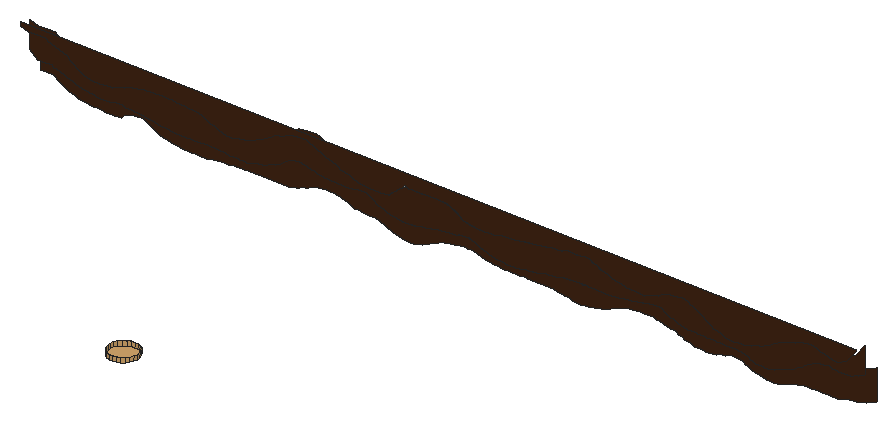
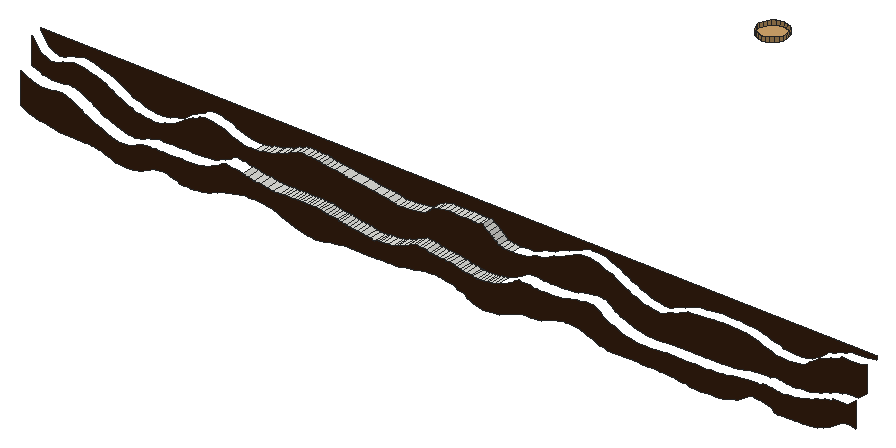
# SketchUp Ruby script. Lengths in inches.
U = 1.inch
M = Sketchup.active_model
def pt(a) = Geom::Point3d.new(a.map { |v| v * U })
def face(e, loops, mat)
  f = e.add_face(loops[0].map { |a| pt(a) })
  loops[1..].each { |l| e.add_face(l.map { |a| pt(a) }).erase! }
  f.material = f.back_material = mat if mat
  f
end
# faces: each face lists its corners as indices into pts; further lists are holes
def faces(e, pts, list, mat = nil) = list.each { |f| face(e, (f[0].is_a?(Array) ? f : [f]).map { |l| l.map { |i| pts[i] } }, mat) }
# xy, xz, yz: faces in a plane at the given z, y or x. An outline is a flat list of corners, or four numbers for a rectangle; further outlines are holes
def ring(l) = l.size == 4 ? [[l[0], l[1]], [l[2], l[1]], [l[2], l[3]], [l[0], l[3]]] : l.each_slice(2).to_a
def flat(e, list, mat, &to3) = list.each { |f| face(e, (f[0].is_a?(Array) ? f : [f]).map { |l| ring(l).map { |u, v| to3.(u, v) } }, mat) }
def xy(e, z, list, mat = nil) = flat(e, list, mat) { |x, y| [x, y, z] }
def xz(e, y, list, mat = nil) = flat(e, list, mat) { |x, z| [x, y, z] }
def yz(e, x, list, mat = nil) = flat(e, list, mat) { |y, z| [x, y, z] }
def lines(e, pts, list) = list.each { |a, b| e.add_line(pt(pts[a]), pt(pts[b])) }
# prism: a flat outline (further loops are holes) pulled along v
def prism(e, loops, v, mat = nil)
  f = face(e, loops, mat); d = Geom::Vector3d.new(v.map { |x| x * U })
  f.pushpull(f.normal.samedirection?(d) ? d.length : -d.length)
end
def box(e, o, s, mat = nil) = prism(e, [[o, [o[0] + s[0], o[1], o[2]], [o[0] + s[0], o[1] + s[1], o[2]], [o[0], o[1] + s[1], o[2]]]], [0, 0, s[2]], mat)
def at(x, y, z, deg = 0) = Geom::Transformation.translation(pt([x, y, z])) * Geom::Transformation.rotation(ORIGIN, Z_AXIS, deg.degrees)
def axes(o, x, y, z) = Geom::Transformation.new([*x, 0, *y, 0, *z, 0, *pt(o).to_a, 1])
def part(name) = M.definitions.add(name)
# library, detail: a bought-in or finely detailed component or shape, given as its bounding box
def library(name, o, s) = part(name).tap { |d| box(d.entities, o, s) }
def detail(e, o, s) = box(e.add_group.entities, o, s)
def put(e, d, t, mat = nil) = e.add_instance(d, t).tap { |i| i.material = mat if mat }
def group(e, t, mat = nil) = e.add_group.tap { |g| g.transformation = t; g.material = mat if mat }.entities
root = M.entities
M.materials.add("[Field Square Tile]").color = [211, 167, 108]
M.materials.add("[Wood Veneer 01]").color = [66, 38, 20]
xy(root,243.05,[[1237.04,563.18,1237.72,565.74]])
xy(root,243.07,[[1235.1875,563.18,1235.77,565.74]])
xy(root,243.09,[[1231.875,563.18,1232.4,565.74],[1232.4,563.18,1232.92,565.74],[1232.92,563.18,1233.58,565.74],[1233.58,563.18,1234.03,565.74]])
xy(root,249.21,[[1204.67,561.05,1205.56,563.18]])
xy(root,249.22,[[1206.28,561.05,1207.1875,563.18]])
xy(root,249.23,[[1207.83,561.05,1208.73,563.18]])
xy(root,250.6875,[[1203.22,492.77,1202.56,492.86,1201.94,493.11,1201.41,493.52,1201,494.05,1200.75,494.67,1200.66,495.33,1200.75,495.99,1201,496.61,1201.41,497.14,1201.94,497.55,1202.56,497.81,1203.22,497.89,1203.88,497.81,1204.5,497.55,1205.03,497.14,1205.44,496.61,1205.7,495.99,1205.78,495.33,1205.7,494.67,1205.44,494.05,1205.03,493.52,1204.5,493.11,1203.88,492.86]],"[Field Square Tile]")
xz(root,561.05,[[1263.09,244.87,1264,245.01,1264.9375,245.12,1265.7,245.25,1266.46,245.41,1267.09,245.78,1267.89,245.88,1268.6,246.16,1269.2,246.57,1269.99,246.9,1270.59,247.35,1271.26,247.62,1271.85,248.06,1272.61,248.32,1273.72,248.66,1274.5,248.79,1275.36,249.19,1276.03,249.32,1276.96,249.41,1277.81,249.48,1278.56,249.21,1279.2,248.96,1279.9,248.9,1280.7,248.42,1281.41,248.3,1282.12,248.22,1282.9375,248.56,1283.87,249.02,1285.6,251.16,1285.6,251.5,1131.59,251.5,1131.59,250.88,1133.18,250.53,1134.8,250.54,1136.26,250.55,1136.79,250.15,1137.4,249.97,1138.2,249.8,1138.87,249.41,1139.54,249.2,1140.31,249.01,1140.8,248.51,1141.43,248.07,1142.08,247.72,1142.72,247.25,1143.27,246.88,1143.99,246.73,1144.65,246.62,1145.39,246.54,1146.17,246.51,1146.95,246.58,1147.75,246.59,1148.55,246.69,1149.26,247.03,1149.95,247.2,1150.92,247.39,1151.55,247.78,1152.33,247.89,1153.33,248.18,1153.97,248.29,1154.86,248.35,1155.59,248.4,1156.58,248.4375,1157.24,248.46,1158.13,248.47,1158.87,248.48,1159.76,248.49,1160.49,248.39,1161.89,248.28,1162.92,248.15,1163.74,248.11,1164.54,248.08,1165.38,247.66,1166.01,247.46,1166.69,247.08,1167.375,246.94,1168.23,246.66,1168.84,246.35,1169.61,246.05,1170.51,246.13,1171.22,246.29,1172.02,246.41,1172.93,246.55,1173.66,246.92,1174.27,247.12,1174.95,247.31,1175.52,247.71,1176.45,248.03,1177.16,248.46,1177.94,248.82,1178.66,249.37,1179.45,249.5625,1180.35,249.9,1181.27,250.35,1181.93,250.49,1182.74,250.6,1183.76,250.58,1184.4,250.61,1185.02,250.32,1185.71,250.0625,1186.37,249.68,1187.13,249.46,1188.02,248.95,1189.24,248.69,1190.15,248.26,1190.75,247.9,1191.88,247.66,1192.46,247.53,1193.14,247.25,1193.95,246.95,1194.64,246.75,1195.43,246.66,1196.14,246.59,1197.03,246.55,1197.96,246.63,1198.7,246.74,1199.43,246.87,1200.04,247.42,1200.71,247.96,1201.28,248.44,1202.02,248.85,1202.49,249.34,1203.22,249.125,1203.99,249.17,1204.67,249.21,1205.56,249.21,1206.28,249.22,1207.1875,249.22,1207.83,249.23,1208.73,249.23,1209.47,249.24,1210.27,249.14,1210.9,248.82,1211.69,248.54,1212.39,248.04,1213.08,247.48,1213.97,247.29,1214.79,247.15,1215.52,247.05,1216.24,247,1217.15,246.96,1217.875,246.94,1218.79,247.04,1219.85,247.36,1221.03,247.43,1222.68,247.6,1224.66,247.98,1226.86,248.1875,1228.47,248.49,1229.72,248.62,1230.66,248.69,1231.34,248.75,1232,249.09,1232.7,249.18,1233.48,249.13,1234.18,249.17,1234.88,249.18,1235.78,249.29,1236.51,249.21,1237.12,248.8,1237.8125,248.73,1238.59,248.26,1239.29,248.02,1240.09,247.8125,1240.8,247.4,1241.71,247.27,1242.45,247.18,1243.375,246.91,1244.24,246.84,1245.19,246.79,1245.97,246.75,1246.72,246.83,1247.76,247.25,1248.63,247.55,1249.3,247.66,1249.93,248.16,1250.72,248.41,1251.42,248.52,1252.12,248.72,1252.82,248.8,1253.71,248.85,1254.54,248.6875,1255.08,248.26,1255.77,248.06,1256.66,247.55,1257.37,247.19,1258.18,246.63,1258.8125,246.13,1259.4,245.83,1260.08,245.67,1260.95,245.46,1261.66,245.0625,1262.375,244.95]],"[Wood Veneer 01]")
xz(root,563.18,[[1267.09,241.09,1267.66,241.14,1268.3,241.35,1268.89,241.46,1269.83,241.85,1270.83,242.23,1271.39,242.42,1272.11,242.61,1272.625,242.91,1273,243.14,1273.54,243.52,1274.02,243.71,1274.35,244.02,1274.79,244.21,1275.38,244.57,1275.85,244.76,1276.47,245.125,1276.97,245.32,1277.45,245.41,1278,245.48,1278.49,245.59,1279.02,245.55,1279.63,245.35,1280.12,245.31,1280.67,245.27,1281.23,245.24,1281.79,245.22,1282.35,245.34,1282.98,245.42,1283.5625,245.52,1283.94,245.76,1284.41,245.9,1285.6,246.43,1285.6,251.16,1283.87,249.02,1282.9375,248.56,1282.12,248.22,1281.41,248.3,1280.7,248.42,1279.9,248.9,1279.2,248.96,1278.56,249.21,1277.81,249.48,1276.96,249.41,1276.03,249.32,1275.36,249.19,1274.5,248.79,1273.72,248.66,1272.61,248.32,1271.85,248.06,1271.26,247.62,1270.59,247.35,1269.99,246.9,1269.2,246.57,1268.6,246.16,1267.89,245.88,1267.09,245.78,1266.46,245.41,1265.7,245.25,1264.9375,245.12,1264,245.01,1263.09,244.87,1262.375,244.95,1261.66,245.0625,1260.95,245.46,1260.08,245.67,1259.4,245.83,1258.8125,246.13,1258.18,246.63,1257.37,247.19,1256.66,247.55,1255.77,248.06,1255.08,248.26,1254.54,248.6875,1253.71,248.85,1252.82,248.8,1252.12,248.72,1251.42,248.52,1250.72,248.41,1249.93,248.16,1249.3,247.66,1248.63,247.55,1247.76,247.25,1246.72,246.83,1245.97,246.75,1245.19,246.79,1244.24,246.84,1243.375,246.91,1242.45,247.18,1241.71,247.27,1240.8,247.4,1240.09,247.8125,1239.29,248.02,1238.59,248.26,1237.8125,248.73,1237.12,248.8,1236.51,249.21,1235.78,249.29,1234.88,249.18,1234.18,249.17,1233.48,249.13,1232.7,249.18,1232,249.09,1231.34,248.75,1230.66,248.69,1229.72,248.62,1228.47,248.49,1226.86,248.1875,1224.66,247.98,1222.68,247.6,1221.03,247.43,1219.85,247.36,1218.79,247.04,1217.875,246.94,1217.15,246.96,1216.24,247,1215.52,247.05,1214.79,247.15,1213.97,247.29,1213.08,247.48,1212.39,248.04,1211.69,248.54,1210.9,248.82,1210.27,249.14,1209.47,249.24,1208.73,249.23,1207.83,249.23,1207.1875,249.22,1206.28,249.22,1205.56,249.21,1204.67,249.21,1203.99,249.17,1203.22,249.125,1202.49,249.34,1202.02,248.85,1201.28,248.44,1200.71,247.96,1200.04,247.42,1199.43,246.87,1198.7,246.74,1197.96,246.63,1197.03,246.55,1196.14,246.59,1195.43,246.66,1194.64,246.75,1193.95,246.95,1193.14,247.25,1192.46,247.53,1191.88,247.66,1190.75,247.9,1190.15,248.26,1189.24,248.69,1188.02,248.95,1187.13,249.46,1186.37,249.68,1185.71,250.0625,1185.02,250.32,1184.4,250.61,1183.76,250.58,1182.74,250.6,1181.93,250.49,1181.27,250.35,1180.35,249.9,1179.45,249.5625,1178.66,249.37,1177.94,248.82,1177.16,248.46,1176.45,248.03,1175.52,247.71,1174.95,247.31,1174.27,247.12,1173.66,246.92,1172.93,246.55,1172.02,246.41,1171.22,246.29,1170.51,246.13,1169.61,246.05,1168.84,246.35,1168.23,246.66,1167.375,246.94,1166.69,247.08,1166.01,247.46,1165.38,247.66,1164.54,248.08,1163.74,248.11,1162.92,248.15,1161.89,248.28,1160.49,248.39,1159.76,248.49,1158.87,248.48,1158.13,248.47,1157.24,248.46,1156.58,248.4375,1155.59,248.4,1154.86,248.35,1153.97,248.29,1153.33,248.18,1152.33,247.89,1151.55,247.78,1150.92,247.39,1149.95,247.2,1149.26,247.03,1148.55,246.69,1147.75,246.59,1146.95,246.58,1146.17,246.51,1145.39,246.54,1144.65,246.62,1143.99,246.73,1143.27,246.88,1142.72,247.25,1142.08,247.72,1141.43,248.07,1140.8,248.51,1140.31,249.01,1139.54,249.2,1138.87,249.41,1138.2,249.8,1137.4,249.97,1136.79,250.15,1136.26,250.55,1134.8,250.54,1133.18,250.53,1131.59,250.88,1131.59,246.2,1133.16,244.96,1134.55,244.9375,1135.8,244.92,1136.02,244.61,1136.58,244.54,1137.34,244.41,1138.01,244.11,1138.53,243.95,1139.19,243.79,1139.71,243.48,1140.35,243.3,1140.9375,243.14,1141.42,243.06,1142.14,242.85,1142.72,242.78,1143.53,242.73,1144.07,242.68,1144.74,242.51,1145.26,242.46,1145.8,242.58,1146.43,242.57,1147.06,242.81,1147.63,242.86,1148.19,242.89,1148.83,242.92,1149.26,242.625,1149.87,242.65,1150.42,242.62,1151.05,242.58,1151.61,242.57,1152.25,242.48,1152.91,242.38,1153.57,242.34,1154.24,242.24,1155.41,241.96,1156.18,241.89,1157,241.83,1157.6,241.78,1158.37,241.75,1158.82,241.74,1159.37,241.72,1160.63,241.7,1161.36,241.69,1162.03,241.68,1162.62,241.68,1163.11,241.67,1163.8125,241.74,1164.38,241.75,1166.38,241.75,1166.87,241.67,1167.4,241.66,1168.01,241.57,1168.55,241.53,1169.17,241.51,1169.72,241.49,1170.42,241.48,1171.08,241.47,1171.65,241.46,1172.36,241.6,1173.09,241.85,1173.76,241.91,1174.66,242.1,1175.43,242.46,1176.13,242.78,1176.9,242.97,1177.43,243.23,1177.83,243.48,1178.35,243.72,1178.6875,244.12,1179.16,244.39,1179.64,244.73,1180.125,244.87,1180.71,244.95,1181.39,245.01,1182.04,244.81,1182.61,244.7,1183.09,244.67,1183.7,244.55,1184.24,244.51,1184.7,244.25,1185.45,244.11,1186.01,244.04,1186.63,243.99,1187.35,243.95,1187.85,243.93,1188.54,243.91,1189.11,243.89,1189.81,243.88,1190.46,243.94,1191.1,243.95,1191.66,244.1,1192.29,244.13,1192.77,244.15,1193.29,244.17,1193.81,244.18,1194.41,243.8,1194.95,243.43,1195.56,243.09,1195.95,242.875,1196.45,242.68,1197.04,242.51,1197.55,242.21,1198.15,242.11,1198.83,241.96,1199.39,241.89,1199.85,241.85,1200.37,241.8125,1200.88,241.79,1201.46,241.78,1202.13,241.91,1202.6,241.93,1203.27,242.09,1204.04,242.2,1204.54,242.24,1205.15,242.42,1205.7,242.47,1206.45,242.71,1207.09,242.78,1207.57,242.82,1208.26,242.85,1208.96,242.87,1209.51,243.02,1210.13,243.05,1210.68,243.29,1211.36,243.35,1211.91,243.39,1212.51,243.42,1213.28,243.14,1213.85,242.9375,1214.4,242.65,1215.02,242.39,1215.78,242.14,1216.42,241.89,1216.91,241.78,1217.96,241.63,1218.73,241.56,1219.33,241.51,1219.78,241.48,1220.3,241.46,1221.17,241.51,1221.89,241.59,1222.83,241.82,1223.61,241.87,1224.375,241.98,1224.99,242.02,1225.64,242.19,1226.34,242.38,1226.83,242.4375,1227.35,242.48,1228.01,242.58,1228.54,242.61,1229.125,242.77,1229.58,242.95,1230.14,243.01,1230.65,243.05,1231.22,243.08,1231.875,243.09,1234.03,243.09,1234.6,243.08,1235.1875,243.07,1235.77,243.07,1236.43,243.0625,1237.04,243.05,1237.72,243.05,1238.99,243.1,1240.16,243.17,1241.3,243.4,1242.5625,243.52,1243.69,243.71,1244.59,243.99,1245.29,244.08,1245.99,244.21,1246.57,244.27,1247.11,244.3,1247.78,244.39,1248.375,244.19,1248.75,243.88,1249.23,243.59,1249.78,243.33,1250.33,243.22,1250.82,242.92,1251.3,242.75,1251.86,242.6,1252.42,242.52,1252.98,242.47,1253.5625,242.43,1254.14,242.4,1254.72,242.39,1255.3,242.37,1255.88,242.36,1256.47,242.35,1257.63,242.33,1258.21,242.33,1258.93,242.32,1259.4,242.3125,1260.04,242.3,1260.71,242.3,1261.16,242.29,1261.8,242.28,1262.3125,242.28,1262.94,242.2,1263.52,241.97,1264.09,241.84,1264.6,241.57,1265.02,241.33,1265.49,241.24,1266.02,241.17,1266.49,241.12]],"[Wood Veneer 01]")
xz(root,565.74,[[1200.45,236.98,1201.13,237.22,1201.98,237.43,1202.6,237.74,1203.3,238.02,1203.74,238.375,1204.3,238.51,1204.9375,238.76,1205.58,239.12,1206.16,239.22,1207.16,239.31,1207.97,239.54,1208.46,239.6,1209.08,239.65,1209.67,239.69,1210.23,239.7,1210.96,239.72,1211.57,239.56,1212.24,239.44,1213.09,239.16,1213.64,239.07,1214.41,238.93,1215.29,238.78,1215.77,238.73,1216.44,238.6875,1217.13,238.66,1217.8,238.65,1218.58,238.64,1219.2,238.63,1219.89,238.625,1220.75,238.625,1221.31,238.62,1226.2,238.62,1226.89,238.45,1227.65,238.25,1228.27,238.19,1229.04,238.15,1229.67,237.86,1230.44,237.79,1231.15,237.74,1232.02,237.87,1232.67,237.88,1233.79,238.14,1235.01,238.46,1235.76,238.72,1236.64,239.08,1237.43,239.375,1238.17,239.75,1238.82,239.97,1239.44,240.17,1240.12,240.27,1240.8,240.33,1241.49,240.37,1242.18,240.4,1242.875,240.41,1243.4,240.42,1243.98,240.43,1244.55,240.43,1245.2,240.27,1245.78,240.23,1246.43,239.96,1247.1875,239.8,1247.8,239.65,1248.5625,239.5,1249.1875,239.18,1249.87,239.01,1250.39,238.67,1250.96,238.56,1251.62,238.48,1252.1875,238.26,1252.76,238.19,1253.58,238.15,1254.11,238.11,1254.78,238.18,1255.46,238.18,1256.14,238.27,1256.66,238.55,1257.32,238.61,1257.91,238.66,1258.48,239.04,1259.22,239.125,1259.9,239.02,1260.59,238.96,1261.11,238.86,1261.61,238.57,1262.16,238.33,1262.87,238,1263.7,237.71,1264.24,237.59,1264.84,237.51,1265.43,237.45,1266,237.42,1266.73,237.4,1267.41,237.47,1268.01,237.5625,1268.7,237.84,1269.38,238.08,1270.07,238.33,1270.6,238.51,1271.17,238.6,1271.83,238.74,1272.41,238.8,1272.98,238.83,1273.72,238.86,1274.48,238.875,1275.02,238.88,1275.7,238.89,1276.38,238.89,1277.14,238.9,1278.53,238.9,1279.16,239.15,1279.93,239.28,1280.73,239.42,1281.45,239.49,1282,239.53,1282.6875,239.81,1283.21,239.96,1283.77,240.1,1285.6,240.89,1285.6,246.43,1284.41,245.9,1283.94,245.76,1283.5625,245.52,1282.98,245.42,1282.35,245.34,1281.79,245.22,1281.23,245.24,1280.67,245.27,1280.12,245.31,1279.63,245.35,1279.02,245.55,1278.49,245.59,1278,245.48,1277.45,245.41,1276.97,245.32,1276.47,245.125,1275.85,244.76,1275.38,244.57,1274.79,244.21,1274.35,244.02,1274.02,243.71,1273.54,243.52,1273,243.14,1272.625,242.91,1272.11,242.61,1271.39,242.42,1270.83,242.23,1269.83,241.85,1268.89,241.46,1268.3,241.35,1267.66,241.14,1267.09,241.09,1266.49,241.12,1266.02,241.17,1265.49,241.24,1265.02,241.33,1264.6,241.57,1264.09,241.84,1263.52,241.97,1262.94,242.2,1262.3125,242.28,1261.8,242.28,1261.16,242.29,1260.71,242.3,1260.04,242.3,1259.4,242.3125,1258.93,242.32,1258.21,242.33,1257.63,242.33,1256.47,242.35,1255.88,242.36,1255.3,242.37,1254.72,242.39,1254.14,242.4,1253.5625,242.43,1252.98,242.47,1252.42,242.52,1251.86,242.6,1251.3,242.75,1250.82,242.92,1250.33,243.22,1249.78,243.33,1249.23,243.59,1248.75,243.88,1248.375,244.19,1247.78,244.39,1247.11,244.3,1246.57,244.27,1245.99,244.21,1245.29,244.08,1244.59,243.99,1243.69,243.71,1242.5625,243.52,1241.3,243.4,1240.16,243.17,1238.99,243.1,1237.72,243.05,1237.04,243.05,1236.43,243.0625,1235.77,243.07,1235.1875,243.07,1234.6,243.08,1234.03,243.09,1231.875,243.09,1231.22,243.08,1230.65,243.05,1230.14,243.01,1229.58,242.95,1229.125,242.77,1228.54,242.61,1228.01,242.58,1227.35,242.48,1226.83,242.4375,1226.34,242.38,1225.64,242.19,1224.99,242.02,1224.375,241.98,1223.61,241.87,1222.83,241.82,1221.89,241.59,1221.17,241.51,1220.3,241.46,1219.78,241.48,1219.33,241.51,1218.73,241.56,1217.96,241.63,1216.91,241.78,1216.42,241.89,1215.78,242.14,1215.02,242.39,1214.4,242.65,1213.85,242.9375,1213.28,243.14,1212.51,243.42,1211.91,243.39,1211.36,243.35,1210.68,243.29,1210.13,243.05,1209.51,243.02,1208.96,242.87,1208.26,242.85,1207.57,242.82,1207.09,242.78,1206.45,242.71,1205.7,242.47,1205.15,242.42,1204.54,242.24,1204.04,242.2,1203.27,242.09,1202.6,241.93,1202.13,241.91,1201.46,241.78,1200.88,241.79,1200.37,241.8125,1199.85,241.85,1199.39,241.89,1198.83,241.96,1198.15,242.11,1197.55,242.21,1197.04,242.51,1196.45,242.68,1195.95,242.875,1195.56,243.09,1194.95,243.43,1194.41,243.8,1193.81,244.18,1193.29,244.17,1192.77,244.15,1192.29,244.13,1191.66,244.1,1191.1,243.95,1190.46,243.94,1189.81,243.88,1189.11,243.89,1188.54,243.91,1187.85,243.93,1187.35,243.95,1186.63,243.99,1186.01,244.04,1185.45,244.11,1184.7,244.25,1184.24,244.51,1183.7,244.55,1183.09,244.67,1182.61,244.7,1182.04,244.81,1181.39,245.01,1180.71,244.95,1180.125,244.87,1179.64,244.73,1179.16,244.39,1178.6875,244.12,1178.35,243.72,1177.83,243.48,1177.43,243.23,1176.9,242.97,1176.13,242.78,1175.43,242.46,1174.66,242.1,1173.76,241.91,1173.09,241.85,1172.36,241.6,1171.65,241.46,1171.08,241.47,1170.42,241.48,1169.72,241.49,1169.17,241.51,1168.55,241.53,1168.01,241.57,1167.4,241.66,1166.87,241.67,1166.38,241.75,1164.38,241.75,1163.8125,241.74,1163.11,241.67,1162.62,241.68,1162.03,241.68,1161.36,241.69,1160.63,241.7,1159.37,241.72,1158.82,241.74,1158.37,241.75,1157.6,241.78,1157,241.83,1156.18,241.89,1155.41,241.96,1154.24,242.24,1153.57,242.34,1152.91,242.38,1152.25,242.48,1151.61,242.57,1151.05,242.58,1150.42,242.62,1149.87,242.65,1149.26,242.625,1148.83,242.92,1148.19,242.89,1147.63,242.86,1147.06,242.81,1146.43,242.57,1145.8,242.58,1145.26,242.46,1144.74,242.51,1144.07,242.68,1143.53,242.73,1142.72,242.78,1142.14,242.85,1141.42,243.06,1140.9375,243.14,1140.35,243.3,1139.71,243.48,1139.19,243.79,1138.53,243.95,1138.01,244.11,1137.34,244.41,1136.58,244.54,1136.02,244.61,1135.8,244.92,1134.55,244.9375,1133.16,244.96,1131.59,246.2,1131.59,241.52,1132.8,241.69,1134.07,241.55,1135.09,240.85,1135.63,240.59,1136.23,240.2,1137.02,239.86,1137.47,239.64,1138.03,239.52,1138.54,239.19,1139.32,239.09,1140.01,239.03,1140.69,238.97,1141.39,238.94,1142.09,238.93,1142.78,238.92,1143.82,238.82,1144.33,238.8,1145.2,238.79,1145.94,238.77,1146.47,238.9375,1147.03,239.55,1147.61,239.69,1148.16,239.88,1148.89,239.99,1149.48,240.05,1150.14,240.09,1150.83,240.11,1151.53,239.71,1151.99,239.38,1152.57,239.11,1153.15,238.74,1153.8,238.43,1154.71,238.31,1155.18,238.21,1156.12,237.9,1156.78,237.82,1157.47,237.76,1158.18,237.71,1158.79,237.68,1159.39,237.67,1160.14,237.66,1160.83,237.65,1162.14,237.65,1162.81,237.89,1163.57,237.94,1164.1875,237.98,1165.04,238.1,1165.59,238.13,1166.35,238.15,1166.98,238.26,1167.73,238.28,1168.36,238.3,1169.21,238.32,1169.93,238.33,1171.16,238.33,1171.84,238.34,1177.41,238.34,1177.92,238.59,1178.74,238.72,1179.43,238.86,1179.94,239.18,1180.53,239.35,1181.09,239.52,1181.64,239.85,1182.28,240.03,1182.9375,240.12,1183.61,240.19,1184.375,240.23,1185.08,240.25,1185.7,240.27,1186.48,240.11,1187.11,239.92,1187.8,239.7,1188.33,239.53,1188.91,239.29,1189.57,239.04,1190.15,238.94,1190.72,238.875,1191.47,238.83,1192.23,238.8,1192.77,238.79,1193.44,238.78,1194.22,238.43,1195,238.28,1195.5625,237.96,1196.5,237.68,1197.17,237.33,1197.7,237.2,1198.39,237.11,1199.15,237.04,1199.84,237.01]],"[Wood Veneer 01]")
p = [[1218.73,563.18,241.56],[1218.73,565.74,241.56],[1219.33,565.74,241.51],[1219.33,563.18,241.51],[1219.78,565.74,241.48],[1219.78,563.18,241.48],
  [1220.3,565.74,241.46],[1220.3,563.18,241.46],[1221.17,565.74,241.51],[1221.17,563.18,241.51],[1221.89,565.74,241.59],[1221.89,563.18,241.59],
  [1216.91,563.18,241.78],[1216.91,565.74,241.78],[1217.96,565.74,241.63],[1217.96,563.18,241.63],[1222.83,565.74,241.82],[1222.83,563.18,241.82],
  [1199.39,563.18,241.89],[1199.39,565.74,241.89],[1199.85,565.74,241.85],[1199.85,563.18,241.85],[1200.37,565.74,241.8125],[1200.37,563.18,241.8125],
  [1200.88,565.74,241.79],[1200.88,563.18,241.79],[1201.46,565.74,241.78],[1201.46,563.18,241.78],[1202.13,565.74,241.91],[1202.13,563.18,241.91],
  [1216.42,563.18,241.89],[1216.42,565.74,241.89],[1223.61,565.74,241.87],[1223.61,563.18,241.87],[1198.83,563.18,241.96],[1198.83,565.74,241.96],
  [1202.6,565.74,241.93],[1202.6,563.18,241.93],[1203.27,565.74,242.09],[1203.27,563.18,242.09],[1215.78,563.18,242.14],[1215.78,565.74,242.14],
  [1224.375,565.74,241.98],[1224.375,563.18,241.98],[1198.15,563.18,242.11],[1198.15,565.74,242.11],[1224.99,565.74,242.02],[1224.99,563.18,242.02],
  [1225.64,565.74,242.19],[1225.64,563.18,242.19],[1197.55,563.18,242.21],[1197.55,565.74,242.21],[1204.04,565.74,242.2],[1204.04,563.18,242.2],
  [1215.02,563.18,242.39],[1215.02,565.74,242.39],[1204.54,565.74,242.24],[1204.54,563.18,242.24],[1205.15,565.74,242.42],[1205.15,563.18,242.42],
  [1226.34,565.74,242.38],[1226.34,563.18,242.38],[1205.7,565.74,242.47],[1205.7,563.18,242.47],[1214.4,563.18,242.65],[1214.4,565.74,242.65],
  [1226.83,565.74,242.4375],[1226.83,563.18,242.4375],[1227.35,565.74,242.48],[1227.35,563.18,242.48],[1206.45,565.74,242.71],[1206.45,563.18,242.71],
  [1228.01,565.74,242.58],[1228.01,563.18,242.58],[1213.85,563.18,242.9375],[1213.85,565.74,242.9375],[1228.54,565.74,242.61],[1228.54,563.18,242.61],
  [1229.125,565.74,242.77],[1229.125,563.18,242.77],[1207.09,565.74,242.78],[1207.09,563.18,242.78],[1207.57,565.74,242.82],[1207.57,563.18,242.82],
  [1208.26,565.74,242.85],[1208.26,563.18,242.85],[1229.58,565.74,242.95],[1229.58,563.18,242.95],[1208.96,565.74,242.87],[1208.96,563.18,242.87],
  [1209.51,565.74,243.02],[1209.51,563.18,243.02],[1213.28,563.18,243.14],[1213.28,565.74,243.14],[1210.13,565.74,243.05],[1210.13,563.18,243.05],
  [1230.14,565.74,243.01],[1230.14,563.18,243.01],[1230.65,565.74,243.05],[1230.65,563.18,243.05],[1231.22,565.74,243.08],[1231.22,563.18,243.08],
  [1237.72,563.18,243.05],[1237.72,565.74,243.05],[1238.99,565.74,243.1],[1238.99,563.18,243.1],[1210.68,565.74,243.29],[1210.68,563.18,243.29],
  [1212.51,563.18,243.42],[1212.51,565.74,243.42],[1231.875,565.74,243.09],[1231.875,563.18,243.09],[1234.03,563.18,243.09],[1234.03,565.74,243.09],
  [1234.6,565.74,243.08],[1234.6,563.18,243.08],[1235.1875,565.74,243.07],[1235.1875,563.18,243.07],[1235.77,563.18,243.07],[1235.77,565.74,243.07],
  [1236.43,565.74,243.0625],[1236.43,563.18,243.0625],[1237.04,565.74,243.05],[1237.04,563.18,243.05],[1240.16,565.74,243.17],[1240.16,563.18,243.17],
  [1241.3,565.74,243.4],[1241.3,563.18,243.4],[1211.36,565.74,243.35],[1211.36,563.18,243.35],[1211.91,565.74,243.39],[1211.91,563.18,243.39],
  [1242.5625,565.74,243.52],[1242.5625,563.18,243.52],[1243.69,565.74,243.71],[1243.69,563.18,243.71],[1244.59,565.74,243.99],[1244.59,563.18,243.99],
  [1197.03,561.05,246.55],[1197.03,563.18,246.55],[1197.96,563.18,246.63],[1197.96,561.05,246.63],[1198.7,563.18,246.74],[1198.7,561.05,246.74],
  [1199.43,563.18,246.87],[1199.43,561.05,246.87],[1243.375,561.05,246.91],[1243.375,563.18,246.91],[1244.24,563.18,246.84],[1244.24,561.05,246.84],
  [1200.04,563.18,247.42],[1200.04,561.05,247.42],[1217.15,561.05,246.96],[1217.15,563.18,246.96],[1217.875,563.18,246.94],[1217.875,561.05,246.94],
  [1218.79,563.18,247.04],[1218.79,561.05,247.04],[1242.45,561.05,247.18],[1242.45,563.18,247.18],[1214.79,561.05,247.15],[1214.79,563.18,247.15],
  [1215.52,563.18,247.05],[1215.52,561.05,247.05],[1216.24,563.18,247],[1216.24,561.05,247],[1219.85,563.18,247.36],[1219.85,561.05,247.36],
  [1213.97,561.05,247.29],[1213.97,563.18,247.29],[1241.71,561.05,247.27],[1241.71,563.18,247.27],[1213.08,561.05,247.48],[1213.08,563.18,247.48],
  [1240.8,561.05,247.4],[1240.8,563.18,247.4],[1200.71,563.18,247.96],[1200.71,561.05,247.96],[1221.03,563.18,247.43],[1221.03,561.05,247.43],
  [1222.68,563.18,247.6],[1222.68,561.05,247.6],[1240.09,561.05,247.8125],[1240.09,563.18,247.8125],[1212.39,561.05,248.04],[1212.39,563.18,248.04],
  [1224.66,563.18,247.98],[1224.66,561.05,247.98],[1239.29,561.05,248.02],[1239.29,563.18,248.02],[1201.28,563.18,248.44],[1201.28,561.05,248.44],
  [1211.69,561.05,248.54],[1211.69,563.18,248.54],[1226.86,563.18,248.1875],[1226.86,561.05,248.1875],[1238.59,561.05,248.26],[1238.59,563.18,248.26],
  [1228.47,563.18,248.49],[1228.47,561.05,248.49],[1237.8125,561.05,248.73],[1237.8125,563.18,248.73],[1202.02,563.18,248.85],[1202.02,561.05,248.85],
  [1210.9,561.05,248.82],[1210.9,563.18,248.82],[1229.72,563.18,248.62],[1229.72,561.05,248.62],[1230.66,563.18,248.69],[1230.66,561.05,248.69],
  [1231.34,563.18,248.75],[1231.34,561.05,248.75],[1237.12,561.05,248.8],[1237.12,563.18,248.8],[1210.27,561.05,249.14],[1210.27,563.18,249.14],
  [1232,563.18,249.09],[1232,561.05,249.09],[1236.51,561.05,249.21],[1236.51,563.18,249.21],[1202.49,563.18,249.34],[1202.49,561.05,249.34],
  [1203.22,563.18,249.125],[1203.22,561.05,249.125],[1203.99,563.18,249.17],[1203.99,561.05,249.17],[1209.47,561.05,249.24],[1209.47,563.18,249.24],
  [1232.7,563.18,249.18],[1232.7,561.05,249.18],[1233.48,563.18,249.13],[1233.48,561.05,249.13],[1234.18,563.18,249.17],[1234.18,561.05,249.17],
  [1204.67,563.18,249.21],[1204.67,561.05,249.21],[1205.56,561.05,249.21],[1205.56,563.18,249.21],[1206.28,563.18,249.22],[1206.28,561.05,249.22],
  [1207.1875,561.05,249.22],[1207.1875,563.18,249.22],[1207.83,563.18,249.23],[1207.83,561.05,249.23],[1208.73,561.05,249.23],[1208.73,563.18,249.23],
  [1234.88,563.18,249.18],[1234.88,561.05,249.18],[1235.78,563.18,249.29],[1235.78,561.05,249.29],[1203.22,492.77,251.5],[1202.56,492.86,251.5],
  [1202.56,492.86,250.6875],[1203.22,492.77,250.6875],[1203.88,492.86,251.5],[1203.88,492.86,250.6875],[1201.94,493.11,251.5],[1201.94,493.11,250.6875],
  [1204.5,493.11,251.5],[1204.5,493.11,250.6875],[1201.41,493.52,251.5],[1201.41,493.52,250.6875],[1205.03,493.52,251.5],[1205.03,493.52,250.6875],
  [1201,494.05,251.5],[1201,494.05,250.6875],[1205.44,494.05,251.5],[1205.44,494.05,250.6875],[1200.75,494.67,251.5],[1200.75,494.67,250.6875],
  [1205.7,494.67,251.5],[1205.7,494.67,250.6875],[1200.66,495.33,251.5],[1200.66,495.33,250.6875],[1205.78,495.33,251.5],[1205.78,495.33,250.6875],
  [1200.75,495.99,251.5],[1200.75,495.99,250.6875],[1205.7,495.99,251.5],[1205.7,495.99,250.6875],[1201,496.61,251.5],[1201,496.61,250.6875],
  [1205.44,496.61,251.5],[1205.44,496.61,250.6875],[1201.41,497.14,251.5],[1201.41,497.14,250.6875],[1205.03,497.14,251.5],[1205.03,497.14,250.6875],
  [1201.94,497.55,251.5],[1201.94,497.55,250.6875],[1204.5,497.55,251.5],[1204.5,497.55,250.6875],[1202.56,497.81,251.5],[1202.56,497.81,250.6875],
  [1203.88,497.81,251.5],[1203.88,497.81,250.6875],[1203.22,497.89,251.5],[1203.22,497.89,250.6875]]
faces(root,p,[[0,1,2,3],[3,2,4,5],[5,4,6,7],[7,6,8,9],[9,8,10,11],[12,13,14,15],[15,14,1,0],[11,10,16,17],
  [18,19,20,21],[21,20,22,23],[23,22,24,25],[25,24,26,27],[27,26,28,29],[30,31,13,12],[17,16,32,33],[34,35,19,18],
  [29,28,36,37],[37,36,38,39],[40,41,31,30],[33,32,42,43],[44,45,35,34],[43,42,46,47],[47,46,48,49],[50,51,45,44],
  [39,38,52,53],[54,55,41,40],[53,52,56,57],[57,56,58,59],[49,48,60,61],[59,58,62,63],[64,65,55,54],[61,60,66,67],
  [67,66,68,69],[63,62,70,71],[69,68,72,73],[74,75,65,64],[73,72,76,77],[77,76,78,79],[71,70,80,81],[81,80,82,83],
  [83,82,84,85],[79,78,86,87],[85,84,88,89],[89,88,90,91],[92,93,75,74],[91,90,94,95],[87,86,96,97],[97,96,98,99],
  [99,98,100,101],[102,103,104,105],[95,94,106,107],[108,109,93,92],[101,100,110,111],[112,113,114,115],[115,114,116,117],[118,119,120,121],
  [121,120,122,123],[105,104,124,125],[125,124,126,127],[107,106,128,129],[129,128,130,131],[131,130,109,108],[127,126,132,133],[133,132,134,135],
  [135,134,136,137],[138,139,140,141],[141,140,142,143],[143,142,144,145],[146,147,148,149],[145,144,150,151],[152,153,154,155],[155,154,156,157],
  [158,159,147,146],[160,161,162,163],[163,162,164,165],[165,164,153,152],[157,156,166,167],[168,169,161,160],[170,171,159,158],[172,173,169,168],
  [174,175,171,170],[151,150,176,177],[167,166,178,179],[179,178,180,181],[182,183,175,174],[184,185,173,172],[181,180,186,187],[188,189,183,182],
  [177,176,190,191],[192,193,185,184],[187,186,194,195],[196,197,189,188],[195,194,198,199],[200,201,197,196],[191,190,202,203],[204,205,193,192],
  [199,198,206,207],[207,206,208,209],[209,208,210,211],[212,213,201,200],[214,215,205,204],[211,210,216,217],[218,219,213,212],[203,202,220,221],
  [221,220,222,223],[223,222,224,225],[226,227,215,214],[217,216,228,229],[229,228,230,231],[231,230,232,233],[225,224,234,235],[236,237,238,239],
  [240,241,242,243],[244,245,227,226],[233,232,246,247],[247,246,248,249],[249,248,219,218]])
faces(root,p,[[250,251,252,253],[254,250,253,255],[251,256,257,252],[258,254,255,259],[256,260,261,257],[262,258,259,263],[260,264,265,261],[266,262,263,267],
  [264,268,269,265],[270,266,267,271],[268,272,273,269],[274,270,271,275],[272,276,277,273],[278,274,275,279],[276,280,281,277],[282,278,279,283],
  [280,284,285,281],[286,282,283,287],[284,288,289,285],[290,286,287,291],[288,292,293,289],[294,290,291,295],[292,296,297,293],[296,294,295,297]],"[Field Square Tile]")
